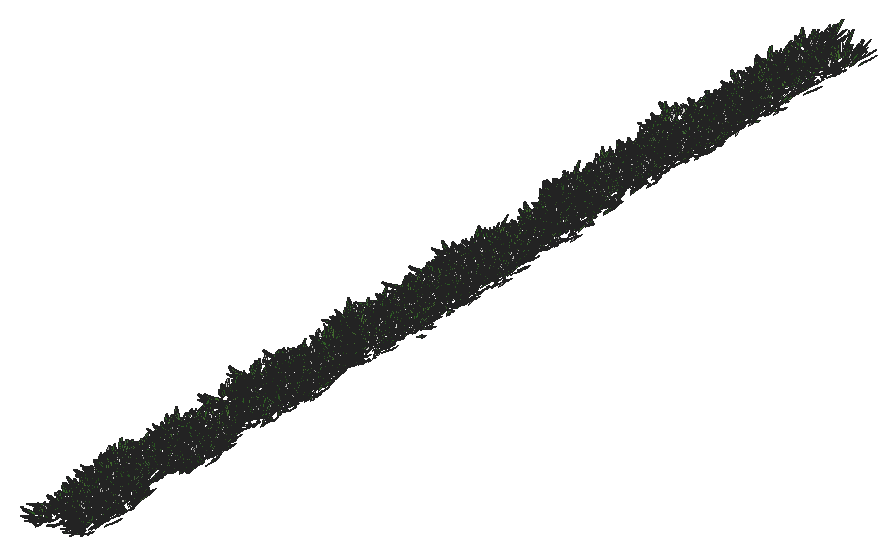
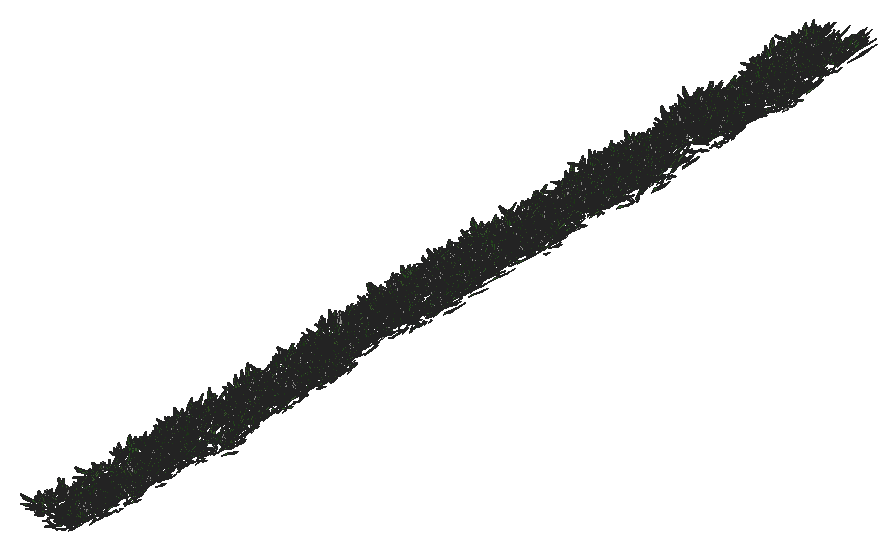
# SketchUp Ruby script. Lengths in inches.
U = 1.inch
M = Sketchup.active_model
def pt(a) = Geom::Point3d.new(a.map { |v| v * U })
def face(e, loops, mat)
  f = e.add_face(loops[0].map { |a| pt(a) })
  loops[1..].each { |l| e.add_face(l.map { |a| pt(a) }).erase! }
  f.material = f.back_material = mat if mat
  f
end
# faces: each face lists its corners as indices into pts; further lists are holes
def faces(e, pts, list, mat = nil) = list.each { |f| face(e, (f[0].is_a?(Array) ? f : [f]).map { |l| l.map { |i| pts[i] } }, mat) }
# xy, xz, yz: faces in a plane at the given z, y or x. An outline is a flat list of corners, or four numbers for a rectangle; further outlines are holes
def ring(l) = l.size == 4 ? [[l[0], l[1]], [l[2], l[1]], [l[2], l[3]], [l[0], l[3]]] : l.each_slice(2).to_a
def flat(e, list, mat, &to3) = list.each { |f| face(e, (f[0].is_a?(Array) ? f : [f]).map { |l| ring(l).map { |u, v| to3.(u, v) } }, mat) }
def xy(e, z, list, mat = nil) = flat(e, list, mat) { |x, y| [x, y, z] }
def xz(e, y, list, mat = nil) = flat(e, list, mat) { |x, z| [x, y, z] }
def yz(e, x, list, mat = nil) = flat(e, list, mat) { |y, z| [x, y, z] }
def lines(e, pts, list) = list.each { |a, b| e.add_line(pt(pts[a]), pt(pts[b])) }
# prism: a flat outline (further loops are holes) pulled along v
def prism(e, loops, v, mat = nil)
  f = face(e, loops, mat); d = Geom::Vector3d.new(v.map { |x| x * U })
  f.pushpull(f.normal.samedirection?(d) ? d.length : -d.length)
end
def box(e, o, s, mat = nil) = prism(e, [[o, [o[0] + s[0], o[1], o[2]], [o[0] + s[0], o[1] + s[1], o[2]], [o[0], o[1] + s[1], o[2]]]], [0, 0, s[2]], mat)
def at(x, y, z, deg = 0) = Geom::Transformation.translation(pt([x, y, z])) * Geom::Transformation.rotation(ORIGIN, Z_AXIS, deg.degrees)
def axes(o, x, y, z) = Geom::Transformation.new([*x, 0, *y, 0, *z, 0, *pt(o).to_a, 1])
def part(name) = M.definitions.add(name)
# library, detail: a bought-in or finely detailed component or shape, given as its bounding box
def library(name, o, s) = part(name).tap { |d| box(d.entities, o, s) }
def detail(e, o, s) = box(e.add_group.entities, o, s)
def put(e, d, t, mat = nil) = e.add_instance(d, t).tap { |i| i.material = mat if mat }
def group(e, t, mat = nil) = e.add_group.tap { |g| g.transformation = t; g.material = mat if mat }.entities
root = M.entities
M.materials.add("Material10").color = [48, 90, 38]
M.materials.add("Material11").color = [68, 110, 48]
M.materials.add("Material12").color = [48, 90, 48]
M.materials.add("Material13").color = [58, 110, 58]
M.materials.add("Material14").color = [58, 90, 38]
M.materials.add("Material15").color = [68, 100, 58]
M.materials.add("Material16").color = [48, 100, 38]
M.materials.add("Material9").color = [68, 110, 58]
c1 = part("grass00")
p = [[-0.6875,0.15,0],[-0.56,0.08,5.52],[-0.04,0.03,2.76],[0.48,-0.02,0],[0.35,-0.02,5.52],[-0.1,-0.14,5.52],
  [-0.12,0.65,8.37],[-0.42,0.65,8.37]]
faces(c1.entities,p,[[0,1,2,3],[3,2,4],[1,5,2],[5,4,2],[1,6,5],[4,5,6],[7,6,1]])
c2 = part("Group16\#1")
put(c2.entities,c1,axes([1.44,-0.61,-0.01],[0.05352,0.12609,0],[-0.10704,0.04543,0.07239],[0.06664,-0.02828,0.11628]),"Material12")
put(c2.entities,c1,axes([0.76,-0.15,-0.01],[0.04676,0.24062,0],[-0.23162,0.04501,0.06642],[0.0652,-0.01267,0.23595]),"Material9")
put(c2.entities,c1,axes([0.79,0.01,-0.01],[-0.00606,0.34651,0],[-0.34381,-0.00602,0.0432],[0.04319,0.00076,0.34386]))
put(c2.entities,c1,axes([1,0.23,-0.01],[-0.07192,0.31144,0],[-0.28722,-0.06632,0.1236],[0.12043,0.02781,0.29478]),"Material11")
put(c2.entities,c1,axes([1.66,0.77,-0.01],[-0.13828,0.29651,0],[-0.21551,-0.1005,0.22471],[0.20365,0.09498,0.23779]),"Material16")
put(c2.entities,c1,axes([0.6875,0.52,-0.01],[-0.18126,0.24051,0],[-0.22746,-0.17142,0.09788],[0.07817,0.05891,0.28481]),"Material11")
put(c2.entities,c1,axes([0.68,0.78,-0.01],[-0.215,0.18688,0],[-0.12385,-0.14248,0.21334],[0.13995,0.16101,0.18878]),"Material9")
put(c2.entities,c1,axes([0.56,1,-0.01],[-0.13756,0.07624,0],[-0.06159,-0.11112,0.0927],[0.04494,0.08108,0.12705]),"Material11")
put(c2.entities,c1,axes([0.2,0.64,-0.01],[-0.23729,0.07254,0],[-0.05711,-0.18681,0.153],[0.04473,0.14632,0.19535]),"Material16")
put(c2.entities,c1,axes([0.0625,0.72,-0.01],[-0.28874,0.02525,0],[-0.02179,-0.24916,0.14647],[0.01276,0.14591,0.25012]),"Material9")
put(c2.entities,c1,axes([-0.08,0.62,-0.01],[-0.34089,-0.04187,0],[0.03255,-0.26504,0.216],[-0.02633,0.21439,0.26703]),"Material16")
put(c2.entities,c1,axes([-0.34,0.98,-0.01],[-0.14314,-0.0493,0],[0.04397,-0.12769,0.06843],[-0.02228,0.0647,0.13505]),"Material16")
put(c2.entities,c1,axes([-0.87,1.45,-0.01],[-0.23488,-0.14114,0],[0.13761,-0.22901,0.06087],[-0.03135,0.05217,0.26717]))
put(c2.entities,c1,axes([-0.72,0.77,-0.01],[-0.14208,-0.13251,0],[0.07209,-0.0773,0.16301],[-0.11118,0.11922,0.1057]),"Material16")
put(c2.entities,c1,axes([-0.62,0.43,-0.01],[-0.14845,-0.21203,0],[0.18654,-0.13061,0.12304],[-0.10079,0.07057,0.22772]),"Material9")
put(c2.entities,c1,axes([-0.68,0.29,-0.01],[-0.13639,-0.32136,0],[0.31723,-0.13464,0.05579],[-0.05136,0.0218,0.34462]),"Material10")
put(c2.entities,c1,axes([-0.64,0.125,-0.01],[-0.0458,-0.23569,0],[0.22124,-0.043,0.08276],[-0.08124,0.01579,0.22538]),"Material13")
put(c2.entities,c1,axes([-1.6,-0.03,-0.01],[0.00576,-0.32897,0],[0.27526,0.00482,0.18018],[-0.18015,-0.00315,0.2753]),"Material11")
put(c2.entities,c1,axes([-1.36,-0.31,-0.01],[0.05718,-0.24765,0],[0.18172,0.04196,0.17267],[-0.16825,-0.03885,0.1865]),"Material16")
put(c2.entities,c1,axes([-1.54,-0.72,-0.01],[0.06537,-0.14017,0],[0.13555,0.06321,0.03939],[-0.0357,-0.01665,0.14956]))
put(c2.entities,c1,axes([-1.19,-0.9,-0.01],[0.09597,-0.12735,0],[0.11214,0.08451,0.07557],[-0.06035,-0.04548,0.14042]),"Material15")
put(c2.entities,c1,axes([-0.47,-0.54,-0.01],[0.11588,-0.10072,0],[0.0618,0.0711,0.12124],[-0.07953,-0.0915,0.0942]))
put(c2.entities,c1,axes([-0.47,-0.84,-0.01],[0.11927,-0.0661,0],[0.06603,0.11913,0.00646],[-0.00313,-0.00565,0.13621]),"Material11")
put(c2.entities,c1,axes([-0.38,-1.24,-0.01],[0.28037,-0.08571,0],[0.0618,0.20215,0.20315],[-0.05939,-0.19428,0.21139]),"Material15")
put(c2.entities,c1,axes([-0.06,-0.66,-0.01],[0.22719,-0.01987,0],[0.01247,0.14255,0.17758],[-0.01547,-0.17691,0.1431]),"Material14")
put(c2.entities,c1,axes([0.11,-0.89,-0.01],[0.14882,0.01828,0],[-0.01058,0.08611,0.12229],[0.01491,-0.12138,0.08676]),"Material12")
put(c2.entities,c1,axes([0.25,-0.72,-0.01],[0.20481,0.07053,0],[-0.06206,0.18022,0.10291],[0.03351,-0.0973,0.1906]),"Material12")
put(c2.entities,c1,axes([0.85,-1.42,-0.01],[0.16481,0.09904,0],[-0.09472,0.15762,0.05616],[0.02893,-0.04814,0.18389]),"Material11")
put(c2.entities,c1,axes([1.01,-1.09,-0.01],[0.21858,0.20385,0],[-0.17495,0.1876,0.15339],[0.10462,-0.11218,0.25652]),"Material16")
put(c2.entities,c1,axes([1.01,-0.71,-0.01],[0.08733,0.12473,0],[-0.06445,0.04512,0.13037],[0.1068,-0.07477,0.07867]),"Material12")
c3 = part("Group15\#1")
put(c3.entities,c2,at(0,0,0))
c4 = part("3darcstudiotree_grass00\#1")
put(c4.entities,c3,at(0,0,0))
put(root,c4,axes([935.98,352.48,12.99],[-0.13459,-6.4522,0],[3.02596,-0.32981,-0.05646],[0.21314,-0.02323,1.57058]))
put(root,c4,axes([935.88,667.21,12.99],[-3.01995,3.34937,0],[-1.50041,-7.06889,-0.06144],[-0.07746,-0.36492,1.3618]))
put(root,c4,axes([934.99,308,12.99],[1.83184,5.03857,0],[-2.3213,4.40976,-0.05468],[-0.16146,0.30672,1.58958]))
put(root,c4,axes([934.97,403.52,12.99],[3.26766,2.6841,0],[-1.08802,6.92121,-0.03831],[-0.04498,0.28615,1.53223]))
put(root,c4,axes([935.52,658.01,12.99],[-1.43456,4.85489,0],[-2.86608,-4.42519,-0.01862],[-0.0613,-0.09465,1.88514]))
put(root,c4,axes([935.7,593.03,12.99],[-0.57031,5.71899,0],[-2.42768,-1.265,-0.03421],[-0.18322,-0.09547,1.87625]))
put(root,c4,axes([935.14,317.33,12.99],[1.72525,6.81797,0],[-2.72996,3.60959,-0.02506],[-0.09165,0.12119,1.82822]))
put(root,c4,axes([936.3,459.02,12.99],[-1.591,4.90781,0],[-2.51291,-4.25661,-0.05517],[-0.17874,-0.30277,1.72999]))
put(root,c4,axes([935.86,383.5625,12.99],[2.25932,4.12484,0],[-1.88326,5.38995,-0.04015],[-0.08457,0.24203,1.39698]))
put(root,c4,axes([937.52,531.4,12.99],[-3.04054,-0.25367,0],[0.11095,-6.9487,-0.04384],[0.0064,-0.40058,1.66887]))
put(root,c4,axes([937.59,720.63,12.99],[1.38326,-7.10685,0],[2.47923,2.52143,-0.03607],[0.12528,0.12741,1.41495]))
put(root,c4,axes([938.31,279.4375,12.99],[-2.71451,-2.68959,0],[0.98077,-5.17223,-0.04544],[0.07965,-0.42002,1.4908]))
put(root,c4,axes([938.13,522.33,12.99],[-2.62733,3.82223,0],[-1.33006,-4.77722,-0.04609],[-0.1244,-0.44681,1.7083]))
put(root,c4,axes([938.5,419.11,12.99],[-3.30552,1.75326,0],[-0.59577,-5.86917,-0.03599],[-0.03233,-0.31848,1.43677]))
put(root,c4,axes([938.65,542.7,12.99],[-1.73136,-4.35948,0],[2.43063,-5.04403,-0.05879],[0.16057,-0.33322,1.66118]))
put(root,c4,axes([937.68,643.52,12.99],[1.88086,4.30043,0],[-1.97027,4.50272,-0.04694],[-0.14738,0.33681,1.69685]))
put(root,c4,axes([937.94,616.88,12.99],[2.70065,-2.14633,0],[0.92371,6.07314,-0.02118],[0.03123,0.20534,1.73224]))
put(root,c4,axes([938.62,511.61,12.99],[-2.62146,1.39695,0],[-0.78385,-7.68601,-0.06463],[-0.04121,-0.40412,1.33032]))
put(root,c4,axes([938.8,598.31,12.99],[-0.21222,-6.92832,0],[3.0608,-0.48989,-0.04142],[0.16952,-0.02713,1.72685]))
put(root,c4,axes([937.83,627.28,12.99],[0.9451,5.56655,0],[-2.97171,2.63636,-0.04732],[-0.14314,0.12699,1.41896]))
put(root,c4,axes([938.54,339.5,12.99],[2.32975,-3.98306,0],[1.99853,6.10813,-0.02614],[0.05074,0.15509,1.48366]))
put(root,c4,axes([939.34,693.84,12.99],[-0.85182,-7.17385,0],[2.69897,-1.67456,-0.0298],[0.10756,-0.06674,1.43464]))
put(root,c4,axes([938.77,306.7,12.99],[-1.58596,5.82577,0],[-2.81489,-4.00411,-0.04897],[-0.17903,-0.25467,1.9584]))
put(root,c4,axes([938.37,292.63,12.99],[2.24371,2.2194,0],[-0.97469,5.14879,-0.02703],[-0.06125,0.32354,1.9211]))
put(root,c4,axes([938.47,607.6,12.99],[2.63039,3.3305,0],[-1.53387,6.33,-0.02111],[-0.04495,0.18549,1.90804]))
put(root,c4,axes([939.83,415.22,12.99],[-2.53383,-3.14385,0],[1.41219,-5.94722,-0.04387],[0.08783,-0.3699,1.70431]))
put(root,c4,axes([938.58,395.41,12.99],[1.13296,5.00949,0],[-2.88403,3.40821,-0.03477],[-0.11779,0.1392,1.69826]))
put(root,c4,axes([938.86,588.54,12.99],[3.13772,0.9132,0],[-0.32035,5.7514,-0.04636],[-0.03117,0.55957,1.85211]))
put(root,c4,axes([939.53,343.8,12.99],[-2.09011,4.78418,0],[-2.14986,-4.9077,-0.05526],[-0.15936,-0.36378,1.69871]))
put(root,c4,axes([939.54,315.5625,12.99],[1.77303,-5.92627,0],[2.1407,3.34653,-0.02882],[0.09506,0.14861,1.42183]))
put(root,c4,axes([939.51,701.92,12.99],[-2.08736,3.58032,0],[-1.98338,-6.04208,-0.02868],[-0.05278,-0.16078,1.39]))
put(root,c4,axes([939.86,505.84,12.99],[0.27846,-6.88397,0],[2.64852,0.5598,-0.04487],[0.17322,0.03661,1.41449]))
put(root,c4,axes([940.16,499.43,12.99],[-3.2612,-0.39296,0],[0.17354,-7.52545,-0.0488],[0.00941,-0.40818,1.65721]))
put(root,c4,axes([940.33,636.66,12.99],[-1.87336,-5.00142,0],[2.3164,-4.53363,-0.03189],[0.08875,-0.17369,1.53238]))
put(root,c4,axes([940.06,265.14,12.99],[-2.56718,0.8353,0],[-0.37583,-6.03536,-0.03826],[-0.02439,-0.39163,1.65468]))
put(root,c4,axes([940.47,483.85,12.99],[-3.15837,-1.26985,0],[0.58083,-7.54849,-0.04722],[0.02497,-0.32447,1.40384]))
put(root,c4,axes([939.48,464.65,12.99],[-0.71465,7.14346,0],[-2.90064,-1.5163,-0.0233],[-0.08807,-0.04604,1.58282]))
put(root,c4,axes([939.74,740.58,12.99],[2.56215,-1.48233,0],[0.77613,7.00966,-0.03471],[0.03796,0.34287,1.93398]))
put(root,c4,axes([940.1,714.11,12.99],[-1.43731,6.01307,0],[-2.9188,-3.64554,-0.04785],[-0.16356,-0.20428,1.77706]))
put(root,c4,axes([939.52,384.59,12.99],[2.80038,4.11369,0],[-1.89207,6.73021,-0.03131],[-0.05251,0.18678,1.48921]))
put(root,c4,axes([939.7,440.29,12.99],[2.00611,6.2173,0],[-2.68637,4.52922,-0.05484],[-0.12668,0.21358,1.31443]))
put(root,c4,axes([939.93,679.67,12.99],[2.90794,1.65532,0],[-0.68554,6.29276,-0.04825],[-0.04373,0.40142,1.45973]))
put(root,c4,axes([940.34,571.26,12.99],[2.42713,0.51867,0],[-0.28756,7.03122,-0.04931],[-0.01666,0.40734,1.538]))
put(root,c4,axes([940.28,456.43,12.99],[0.11465,6.63747,0],[-3.50192,0.31608,-0.04149],[-0.13307,0.01201,1.54325]))
put(root,c4,axes([941.9,402.69,12.99],[-0.5614,-5.61075,0],[3.10386,-1.62278,-0.04627],[0.19246,-0.10063,1.86363]))
put(root,c4,axes([941.93,344.05,12.99],[-3.05629,0.58163,0],[-0.20978,-5.76002,-0.02559],[-0.01195,-0.32822,1.95328]))
put(root,c4,axes([942.5,392.49,12.99],[0.73988,-5.68816,0],[3.2715,2.22351,-0.06029],[0.22067,0.14998,1.78762]))
put(root,c4,axes([942.41,578.12,12.99],[-2.62445,3.8934,0],[-1.496,-5.2692,-0.02727],[-0.05559,-0.19579,1.41127]))
put(root,c4,axes([942.28,483.23,12.99],[1.55628,-5.30455,0],[2.7486,4.21363,-0.05795],[0.20607,0.31591,1.94389]))
put(root,c4,axes([941.8,289.91,12.99],[2.80561,0.69907,0],[-0.2737,5.73969,-0.03498],[-0.01624,0.34054,1.48455]))
put(root,c4,axes([941.82,681.3125,12.99],[2.10378,3.42913,0],[-1.70134,5.45397,-0.03635],[-0.07408,0.23748,1.41103]))
put(root,c4,axes([942.08,599.45,12.99],[0.83053,6.56694,0],[-2.56393,1.69436,-0.04889],[-0.18828,0.12442,1.46761]))
put(root,c4,axes([942.29,271.67,12.99],[0.20148,6.83901,0],[-2.63929,0.40629,-0.04154],[-0.2128,0.03276,1.86323]))
put(root,c4,axes([943.35,431.04,12.99],[-3.33513,-1.5198,0],[0.64635,-7.41133,-0.01918],[0.01574,-0.18048,1.90358]))
put(root,c4,axes([942.44,460.85,12.99],[2.21035,-3.30354,0],[1.35675,4.74337,-0.045],[0.09941,0.34756,1.37282]))
put(root,c4,axes([942.93,745.57,12.99],[1.0169,-5.16651,0],[2.89582,2.97822,-0.04402],[0.16758,0.17235,1.81837]))
put(root,c4,axes([943.22,534.65,12.99],[1.2147,-4.89497,0],[3.03033,3.9293,-0.03953],[0.12753,0.16537,1.77239]))
put(root,c4,axes([943.75,569.58,12.99],[-2.58709,-2.44231,0],[1.06935,-5.91882,-0.04671],[0.08599,-0.47595,1.85324]))
put(root,c4,axes([943.82,737.86,12.99],[-2.41732,-1.12034,0],[0.65586,-7.39435,-0.02938],[0.01703,-0.19204,1.3208]))
put(root,c4,axes([943.05,439.02,12.99],[2.7589,-2.87955,0],[1.3206,6.6113,-0.05401],[0.07416,0.37126,1.44188]))
put(root,c4,axes([943.08,541.3,12.99],[0.676,7.50295,0],[-2.72848,1.28451,-0.03105],[-0.14956,0.07041,1.87912]))
put(root,c4,axes([944.27,495.14,12.99],[-2.69757,-3.22714,0],[1.43513,-6.26832,-0.05348],[0.10735,-0.46886,1.83786]))
put(root,c4,axes([942.85,710.3,12.99],[1.34717,7.13699,0],[-3.06358,3.02162,-0.02206],[-0.0728,0.07181,1.64521]))
put(root,c4,axes([943.27,561.56,12.99],[0.94649,7.45427,0],[-2.44169,1.61997,-0.03743],[-0.14471,0.09601,1.40382]))
put(root,c4,axes([944.41,501.91,12.99],[-3.12121,1.79358,0],[-0.63624,-5.78536,-0.03206],[-0.03576,-0.32519,1.63785]))
put(root,c4,axes([943.64,607.37,12.99],[1.78504,3.9665,0],[-2.26932,5.33631,-0.04673],[-0.10608,0.24945,1.45453]))
put(root,c4,axes([943.96,615.93,12.99],[3.16838,-2.06619,0],[0.95904,7.68441,-0.04256],[0.03786,0.30338,1.55488]))
put(root,c4,axes([943.68,466.74,12.99],[1.81466,4.27064,0],[-2.32191,5.15528,-0.03466],[-0.10632,0.23605,1.89896]))
put(root,c4,axes([943.72,410.54,12.99],[2.57592,3.81949,0],[-1.81471,6.39496,-0.05832],[-0.10338,0.36432,1.48992]))
put(root,c4,axes([944.11,478.1875,12.99],[-0.02884,6.14524,0],[-2.76894,-0.0679,-0.03184],[-0.14375,-0.00352,1.71482]))
put(root,c4,axes([944.39,356.84,12.99],[-1.44175,6.30696,0],[-3.07559,-3.67369,-0.06253],[-0.22087,-0.26382,1.89715]))
put(root,c4,axes([944.21,623.85,12.99],[0.47305,7.00599,0],[-2.58998,0.91377,-0.04631],[-0.21069,0.07433,1.65491]))
put(root,c4,axes([944.11,689.4375,12.99],[0.53759,6.03755,0],[-2.74927,1.27912,-0.02796],[-0.13864,0.0645,1.94708]))
put(root,c4,axes([944.54,633.13,12.99],[0.78201,5.56558,0],[-2.52577,1.85438,-0.04361],[-0.18365,0.13484,1.60948]))
put(root,c4,axes([944.4,722.34,12.99],[2.04517,4.03266,0],[-1.97589,5.23607,-0.02494],[-0.06421,0.17016,1.63549]))
put(root,c4,axes([945.94,402.9,12.99],[-2.6509,-3.28893,0],[1.57343,-6.62659,-0.04044],[0.07948,-0.33474,1.86421]))
put(root,c4,axes([945.75,580.99,12.99],[-0.17778,-5.9494,0],[2.94621,-0.46003,-0.04502],[0.14427,-0.02253,1.30109]))
put(root,c4,axes([946.15,383.4,12.99],[-2.7452,-2.05272,0],[0.78435,-5.48103,-0.035],[0.05446,-0.38057,1.73222]))
put(root,c4,axes([945.9375,308.33,12.99],[-2.42866,3.62409,0],[-1.80185,-6.30944,-0.04574],[-0.1023,-0.35823,1.85022]))
put(root,c4,axes([946.68,418.62,12.99],[-2.24616,-5.29494,0],[2.04559,-4.53423,-0.04714],[0.13743,-0.30462,1.58733]))
put(root,c4,axes([945.64,287.0625,12.99],[3.48632,-0.84276,0],[0.36151,7.81427,-0.02611],[0.01142,0.24694,1.96192]))
put(root,c4,axes([946.59,709.27,12.99],[1.45157,-6.44615,0],[3.03586,3.57211,-0.06088],[0.19233,0.2263,1.6642]))
put(root,c4,axes([947.12,321.27,12.99],[-2.322,-2.26787,0],[1.33389,-7.13622,-0.04539],[0.07371,-0.39432,1.92461]))
put(root,c4,axes([947.07,730.0625,12.99],[-2.53154,-0.11911,0],[0.07095,-7.87949,-0.05231],[0.00434,-0.48228,1.90792]))
put(root,c4,axes([946.17,507.81,12.99],[3.23225,-0.69349,0],[0.28827,7.02045,-0.03728],[0.01567,0.38155,1.90298]))
put(root,c4,axes([946.43,483.95,12.99],[3.12668,-2.99055,0],[1.07667,5.88191,-0.04818],[0.07176,0.39204,1.47658]))
put(root,c4,axes([946.62,479.83,12.99],[2.6073,-0.46987,0],[0.27334,7.92524,-0.03935],[0.00937,0.27166,1.44542]))
put(root,c4,axes([947.16,446.73,12.99],[1.64488,-4.21526,0],[2.41495,4.92407,-0.04874],[0.11803,0.24066,1.44038]))
put(root,c4,axes([946.57,337.22,12.99],[3.2581,-0.00779,0],[0.00346,7.56083,-0.04894],[0.00016,0.34805,1.41164]))
put(root,c4,axes([947.1,636.62,12.99],[-1.24242,7.13984,0],[-2.32471,-2.11374,-0.04072],[-0.16933,-0.15397,1.53595]))
put(root,c4,axes([947.74,667.48,12.99],[-2.32196,-2.16556,0],[1.12319,-6.2928,-0.03312],[0.05955,-0.33364,1.94116]))
put(root,c4,axes([947.09,704.06,12.99],[2.74503,-2.20879,0],[1.1554,7.50291,-0.03514],[0.03813,0.24763,1.55988]))
put(root,c4,axes([946.91,544.74,12.99],[2.52814,4.28272,0],[-1.65787,5.11371,-0.03152],[-0.07249,0.2236,1.47514]))
put(root,c4,axes([948.375,274.15,12.99],[-1.15474,-4.98906,0],[2.56973,-3.10782,-0.0302],[0.11214,-0.13562,1.67548]))
put(root,c4,axes([947.43,595.49,12.99],[2.76462,-1.55361,0],[0.64086,5.95889,-0.02888],[0.03247,0.30194,1.73467]))
put(root,c4,axes([947.65,656.93,12.99],[-0.49517,6.66423,0],[-3.10276,-1.20465,-0.06003],[-0.25304,-0.09824,1.84592]))
put(root,c4,axes([947.39,345.97,12.99],[0.87429,5.2645,0],[-3.22056,2.79469,-0.02635],[-0.08859,0.07688,1.69955]))
put(root,c4,axes([948.62,681.41,12.99],[1.14014,-5.96549,0],[2.97835,2.97436,-0.02716],[0.0819,0.08179,1.46706]))
put(root,c4,axes([948.24,367.23,12.99],[1.97219,-3.26454,0],[1.66188,5.24604,-0.04376],[0.11528,0.36391,1.7457]))
put(root,c4,axes([950.21,296.625,12.99],[-2.83714,-4.55225,0],[1.52377,-4.96226,-0.02484],[0.06516,-0.21221,1.66133]))
put(root,c4,axes([950,517.22,12.99],[-3.04075,1.42126,0],[-0.54404,-6.08193,-0.0347],[-0.0301,-0.33646,1.61275]))
put(root,c4,axes([950.17,639.77,12.99],[-1.46181,-5.17888,0],[2.12491,-3.13401,-0.04434],[0.14176,-0.20908,1.31982]))
put(root,c4,axes([950.34,273.34,12.99],[-2.3144,2.78716,0],[-1.20482,-5.22763,-0.01732],[-0.04346,-0.18859,1.90951]))
put(root,c4,axes([950.4,685.8125,12.99],[-2.10044,4.18736,0],[-1.93703,-5.07707,-0.0546],[-0.1642,-0.43038,1.84968]))
put(root,c4,axes([949.75,545.98,12.99],[0.19711,7.40086,0],[-2.79481,0.38894,-0.02381],[-0.11004,0.01531,1.77807]))
put(root,c4,axes([950.67,587.38,12.99],[0.1657,-6.19204,0],[3.05826,0.42763,-0.05271],[0.17241,0.02411,1.37729]))
put(root,c4,axes([949.8,305.67,12.99],[2.83532,3.44255,0],[-1.26951,5.46339,-0.04207],[-0.10069,0.43333,1.89419]))
put(root,c4,axes([950.5,520.67,12.99],[1.48315,-4.99397,0],[2.04211,3.169,-0.03969],[0.13743,0.21327,1.41714]))
put(root,c4,axes([951.17,573.55,12.99],[-2.10778,-4.99727,0],[1.85456,-4.08732,-0.03577],[0.10883,-0.23986,1.49339]))
put(root,c4,axes([950.11,374.64,12.99],[1.58744,5.33082,0],[-2.10084,3.26891,-0.02533],[-0.09539,0.14843,1.58831]))
put(root,c4,axes([950.33,346.82,12.99],[0.68217,7.65287,0],[-2.98006,1.38804,-0.0503],[-0.18601,0.08664,1.57458]))
put(root,c4,axes([950.26,561.57,12.99],[0.75552,5.6239,0],[-3.03182,2.12822,-0.03259],[-0.12681,0.08902,1.77089]))
put(root,c4,axes([950.26,620.94,12.99],[2.16853,5.2572,0],[-1.8984,4.09169,-0.02839],[-0.10882,0.23454,1.88589]))
put(root,c4,axes([951.36,334.12,12.99],[0.65364,-7.37213,0],[3.23882,1.50051,-0.041],[0.15653,0.07252,1.76588]))
put(root,c4,axes([951.04,675.08,12.99],[2.17217,-4.01041,0],[1.76535,4.99621,-0.03491],[0.1053,0.29801,1.84986]))
put(root,c4,axes([950.48,316.54,12.99],[3.06316,2.08281,0],[-0.89662,6.89021,-0.03162],[-0.02809,0.21587,1.3441]))
put(root,c4,axes([951.54,278.07,12.99],[1.16852,-6.13874,0],[2.70204,2.68754,-0.04597],[0.14491,0.14413,1.38947]))
put(root,c4,axes([952.2,292.28,12.99],[-3.15971,-2.74691,0],[0.94105,-5.65614,-0.04106],[0.06912,-0.41545,1.71966]))
put(root,c4,axes([952.14,507.77,12.99],[-2.28105,3.21822,0],[-1.30075,-4.81745,-0.03387],[-0.07094,-0.26274,1.3548]))
put(root,c4,axes([952.62,443.35,12.99],[-0.55245,-7.53321,0],[2.95971,-1.13415,-0.02808],[0.1128,-0.04322,1.67665]))
put(root,c4,axes([952.52,626.19,12.99],[-2.99233,1.01161,0],[-0.44676,-6.90514,-0.04443],[-0.02837,-0.43843,1.82802]))
put(root,c4,axes([952.0625,362.9375,12.99],[1.75584,-6.75344,0],[2.24087,3.04425,-0.0411],[0.15063,0.20463,1.52451]))
put(root,c4,axes([951.47,420.67,12.99],[2.38201,1.98443,0],[-1.19184,7.4753,-0.03532],[-0.04548,0.28525,1.79519]))
put(root,c4,axes([951.44,532.89,12.99],[2.42536,4.25073,0],[-1.5281,4.55585,-0.03117],[-0.07176,0.21396,1.30357]))
put(root,c4,axes([951.83,396.54,12.99],[0.39276,6.09308,0],[-2.53277,0.85309,-0.04131],[-0.15674,0.05279,1.34689]))
put(root,c4,axes([952.19,358.88,12.99],[2.9137,-4.45489,0],[1.36749,4.67344,-0.03191],[0.09434,0.32241,1.79443]))
put(root,c4,axes([952.45,648.04,12.99],[2.20493,-5.84071,0],[2.17957,4.29937,-0.04774],[0.17483,0.34486,1.91023]))
put(root,c4,axes([952.53,427.9375,12.99],[0.41044,7.34142,0],[-2.57389,0.75191,-0.04145],[-0.22777,0.06654,1.97198]))
put(root,c4,axes([952.48,665.1875,12.99],[2.48522,-0.30078,0],[0.13342,5.76025,-0.02933],[0.00885,0.38213,1.97542]))
put(root,c4,axes([952.35,457.875,12.99],[2.70904,3.83936,0],[-1.48286,5.46714,-0.03504],[-0.09127,0.3365,1.90819]))
put(root,c4,axes([953.99,299.1,12.99],[-0.81569,-6.16766,0],[3.26694,-2.25763,-0.03772],[0.10555,-0.07294,1.36861]))
put(root,c4,axes([954.01,601.8125,12.99],[-2.34471,-3.89429,0],[1.84566,-5.80656,-0.03763],[0.09992,-0.31435,1.94544]))
put(root,c4,axes([954.26,562.34,12.99],[-2.48059,-5.12211,0],[2.14674,-5.4324,-0.0585],[0.17038,-0.43116,1.90866]))
put(root,c4,axes([953.83,427.23,12.99],[-1.63132,4.88764,0],[-2.28424,-3.98369,-0.05103],[-0.17709,-0.30884,1.72023]))
put(root,c4,axes([954.58,675.84,12.99],[-1.80135,-3.90958,0],[2.04323,-4.91918,-0.01822],[0.05759,-0.13866,1.86907]))
put(root,c4,axes([953.82,592.91,12.99],[-0.93165,5.61253,0],[-2.49378,-2.163,-0.03389],[-0.14327,-0.12427,1.65454]))
put(root,c4,axes([954.18,478.78,12.99],[-2.45684,4.80463,0],[-1.99644,-5.33432,-0.05065],[-0.113,-0.30193,1.44592]))
put(root,c4,axes([954.7,516.78,12.99],[-2.51038,-1.6484,0],[0.89656,-7.1345,-0.05258],[0.06005,-0.47784,1.84274]))
put(root,c4,axes([955.06,680.64,12.99],[-2.32533,-5.70985,0],[1.8954,-4.03335,-0.04944],[0.16382,-0.3486,1.60821]))
put(root,c4,axes([954.4,739.27,12.99],[-0.84067,6.69557,0],[-2.40823,-1.57995,-0.04255],[-0.2095,-0.13745,1.76068]))
put(root,c4,axes([955.02,548.72,12.99],[-0.05599,-6.31128,0],[3.24014,-0.15019,-0.05384],[0.16023,-0.00743,1.32332]))
put(root,c4,axes([955.15,382.24,12.99],[-2.34198,-2.88763,0],[1.20392,-5.10203,-0.04409],[0.0893,-0.37842,1.48398]))
put(root,c4,axes([954.97,417.98,12.99],[-3.08231,3.39932,0],[-1.2315,-5.83477,-0.02532],[-0.04648,-0.2202,1.64221]))
put(root,c4,axes([955.05,620.14,12.99],[-2.79455,2.49642,0],[-0.8859,-5.18187,-0.02866],[-0.05883,-0.34408,1.88291]))
put(root,c4,axes([954.2,505.03,12.99],[2.82028,2.06028,0],[-0.84044,6.01143,-0.03842],[-0.05899,0.42193,1.90991]))
put(root,c4,axes([955.62,582.92,12.99],[-2.48511,-3.77064,0],[1.92855,-6.64149,-0.03911],[0.06504,-0.22397,1.43856]))
put(root,c4,axes([955.21,540.61,12.99],[-0.00241,-5.88355,0],[2.5127,-0.00537,-0.0371],[0.1987,-0.00042,1.84609]))
put(root,c4,axes([954.65,352.51,12.99],[2.79152,-3.35181,0],[1.22786,5.34339,-0.02304],[0.05279,0.22975,1.78453]))
put(root,c4,axes([955.1,536.37,12.99],[2.67277,-4.37543,0],[1.97362,6.29954,-0.04389],[0.10575,0.33754,1.92393]))
put(root,c4,axes([955.78,469.09,12.99],[0.46764,-7.5848,0],[3.03006,0.97616,-0.02402],[0.10432,0.03361,1.84088]))
put(root,c4,axes([955.875,269.43,12.99],[-2.51956,1.91082,0],[-0.87651,-6.03903,-0.04681],[-0.05945,-0.40959,1.53984]))
put(root,c4,axes([956.21,691.76,12.99],[-1.48771,-6.94889,0],[3.04376,-3.40501,-0.06506],[0.21491,-0.24041,1.70958]))
put(root,c4,axes([955.42,439.23,12.99],[-0.21435,7.43185,0],[-2.47405,-0.37285,-0.03816],[-0.21833,-0.0329,1.95014]))
put(root,c4,axes([956.125,661.25,12.99],[0.88223,-5.75572,0],[3.20361,2.56584,-0.02001],[0.07198,0.05765,1.77455]))
put(root,c4,axes([954.94,337.43,12.99],[2.17118,5.39514,0],[-2.29779,4.83179,-0.033],[-0.10644,0.22383,1.87715]))
put(root,c4,axes([955.34,728.74,12.99],[-0.71607,6.36246,0],[-3.35809,-1.97481,-0.03008],[-0.10824,-0.06365,1.76703]))
put(root,c4,axes([955.18,646.91,12.99],[2.22412,5.43161,0],[-2.25485,4.8245,-0.05678],[-0.13083,0.27992,1.337]))
put(root,c4,axes([956.53,344.17,12.99],[-0.84845,-6.02584,0],[3.02554,-2.22596,-0.0477],[0.14423,-0.10611,1.385]))
put(root,c4,axes([955.88,526.68,12.99],[2.7853,-1.80702,0],[0.84945,6.84151,-0.03157],[0.03582,0.2885,1.77323]))
put(root,c4,axes([956.82,283.57,12.99],[-1.84744,-4.65579,0],[2.0878,-4.32883,-0.0539],[0.14783,-0.30651,1.43163]))
put(root,c4,axes([955.72,330.82,12.99],[2.57659,2.37854,0],[-1.15107,6.51542,-0.03343],[-0.05601,0.31703,1.88641]))
put(root,c4,axes([956.06,495.96,12.99],[-0.11326,6.3716,0],[-2.63974,-0.24518,-0.03031],[-0.1466,-0.01362,1.75443]))
put(root,c4,axes([955.84,405.34,12.99],[2.44994,2.04607,0],[-1.11968,7.00543,-0.04863],[-0.05811,0.36359,1.5585]))
put(root,c4,axes([956.1,709.07,12.99],[2.61814,-1.1208,0],[0.59376,7.24741,-0.05648],[0.03288,0.40137,1.39957]))
put(root,c4,axes([956.27,655.13,12.99],[1.27268,5.06606,0],[-2.75879,3.62138,-0.0451],[-0.17338,0.22759,1.93445]))
put(root,c4,axes([956.27,390.59,12.99],[3.35577,2.31301,0],[-0.80346,6.09093,-0.04516],[-0.0616,0.46695,1.80387]))
put(root,c4,axes([956.79,446,12.99],[-1.68238,6.29725,0],[-2.84819,-3.976,-0.0342],[-0.10436,-0.14569,1.63693]))
put(root,c4,axes([956.55,375.79,12.99],[2.50121,4.48786,0],[-1.68491,4.90673,-0.02005],[-0.06155,0.17925,1.86077]))
put(root,c4,axes([958.07,494.45,12.99],[0.00822,-6.22775,0],[3.36275,0.0232,-0.03692],[0.12632,0.00087,1.57831]))
put(root,c4,axes([958.3125,400.625,12.99],[-0.95867,-5.15282,0],[2.80964,-2.73135,-0.01791],[0.07476,-0.07268,1.89984]))
put(root,c4,axes([958.35,562.9,12.99],[-1.01353,-5.64232,0],[2.76369,-2.59401,-0.04381],[0.17253,-0.16194,1.74465]))
put(root,c4,axes([958.31,288.27,12.99],[-2.32068,2.12639,0],[-1.1124,-6.34363,-0.04281],[-0.07046,-0.40181,1.81418]))
put(root,c4,axes([958.23,471.42,12.99],[2.30124,-4.66392,0],[2.04512,5.27272,-0.03392],[0.07052,0.18182,1.32537]))
put(root,c4,axes([958.02,740.88,12.99],[2.8068,-0.90346,0],[0.38262,6.21116,-0.04526],[0.03005,0.48787,1.7925]))
put(root,c4,axes([959.05,336.01,12.99],[-2.8885,0.62195,0],[-0.27844,-6.75695,-0.0202],[-0.0091,-0.22079,1.95637]))
put(root,c4,axes([959.15,514.48,12.99],[-0.84473,-7.44112,0],[2.57988,-1.53032,-0.03225],[0.13516,-0.08018,1.58326]))
put(root,c4,axes([958.2,268.39,12.99],[2.689,-0.19784,0],[0.07828,5.55943,-0.04101],[0.00542,0.38505,1.37186]))
